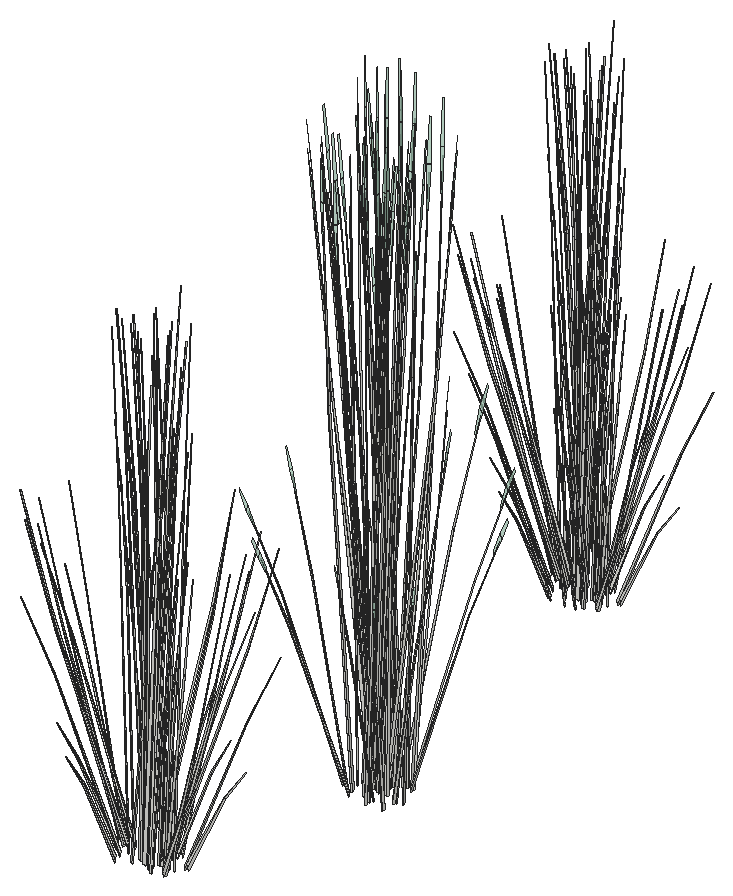
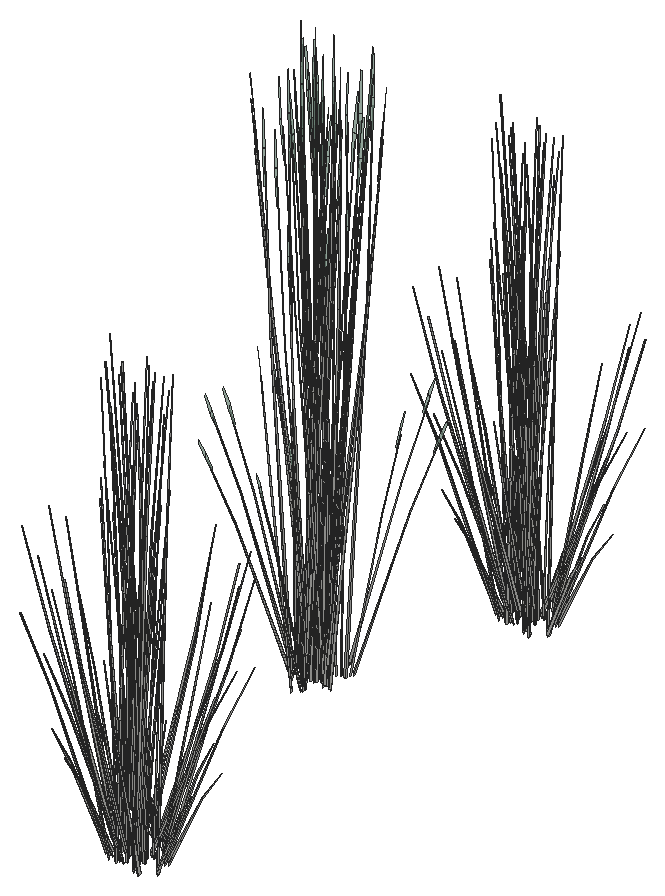
# SketchUp Ruby script. Lengths in inches.
U = 1.inch
M = Sketchup.active_model
def pt(a) = Geom::Point3d.new(a.map { |v| v * U })
def face(e, loops, mat)
  f = e.add_face(loops[0].map { |a| pt(a) })
  loops[1..].each { |l| e.add_face(l.map { |a| pt(a) }).erase! }
  f.material = f.back_material = mat if mat
  f
end
# faces: each face lists its corners as indices into pts; further lists are holes
def faces(e, pts, list, mat = nil) = list.each { |f| face(e, (f[0].is_a?(Array) ? f : [f]).map { |l| l.map { |i| pts[i] } }, mat) }
# xy, xz, yz: faces in a plane at the given z, y or x. An outline is a flat list of corners, or four numbers for a rectangle; further outlines are holes
def ring(l) = l.size == 4 ? [[l[0], l[1]], [l[2], l[1]], [l[2], l[3]], [l[0], l[3]]] : l.each_slice(2).to_a
def flat(e, list, mat, &to3) = list.each { |f| face(e, (f[0].is_a?(Array) ? f : [f]).map { |l| ring(l).map { |u, v| to3.(u, v) } }, mat) }
def xy(e, z, list, mat = nil) = flat(e, list, mat) { |x, y| [x, y, z] }
def xz(e, y, list, mat = nil) = flat(e, list, mat) { |x, z| [x, y, z] }
def yz(e, x, list, mat = nil) = flat(e, list, mat) { |y, z| [x, y, z] }
def lines(e, pts, list) = list.each { |a, b| e.add_line(pt(pts[a]), pt(pts[b])) }
# prism: a flat outline (further loops are holes) pulled along v
def prism(e, loops, v, mat = nil)
  f = face(e, loops, mat); d = Geom::Vector3d.new(v.map { |x| x * U })
  f.pushpull(f.normal.samedirection?(d) ? d.length : -d.length)
end
def box(e, o, s, mat = nil) = prism(e, [[o, [o[0] + s[0], o[1], o[2]], [o[0] + s[0], o[1] + s[1], o[2]], [o[0], o[1] + s[1], o[2]]]], [0, 0, s[2]], mat)
def at(x, y, z, deg = 0) = Geom::Transformation.translation(pt([x, y, z])) * Geom::Transformation.rotation(ORIGIN, Z_AXIS, deg.degrees)
def axes(o, x, y, z) = Geom::Transformation.new([*x, 0, *y, 0, *z, 0, *pt(o).to_a, 1])
def part(name) = M.definitions.add(name)
# library, detail: a bought-in or finely detailed component or shape, given as its bounding box
def library(name, o, s) = part(name).tap { |d| box(d.entities, o, s) }
def detail(e, o, s) = box(e.add_group.entities, o, s)
def put(e, d, t, mat = nil) = e.add_instance(d, t).tap { |i| i.material = mat if mat }
def group(e, t, mat = nil) = e.add_group.tap { |g| g.transformation = t; g.material = mat if mat }.entities
root = M.entities
M.materials.add("LightPink_Translucent").color = [175, 214, 192]
M.materials["LightPink_Translucent"].alpha = 0.75
c1 = part("blade")
p = [[2.15,0.21,22],[0,0.17,0],[0.09,0.45,0],[2.18,0.31,22],[2.29,0.31,22],[0.38,0.45,0],
  [2.48,0.24,33],[2.49,0.24,33],[2.48,0.22,33]]
faces(c1.entities,p,[[0,1,2,3],[4,5,2,3],[6,3,4,7],[8,0,3,6]])
c2 = part("blade with seeds\#1")
put(c2.entities,c1,at(0,0,0))
c3 = part("seeds")
p = [[0.3,-0.1,1.38],[-0.01,-0.03,1.59],[-0.01,-0.03,0.03],[0.14,-0.07,-0.07],[0.29,-0.03,3],[0.15,0.01,3.11]]
faces(c3.entities,p,[[0,1,2,3],[1,0,4,5]],"LightPink_Translucent")
c4 = part("blade with seeds")
put(c4.entities,c1,at(0,0,0))
put(c4.entities,c3,axes([2.4,0.25,30.99],[1.5799,-0.05474,1.17369],[-0.12525,1.92788,0.29478],[-0.07173,-0.02425,1.56792]))
put(root,c2,axes([484.73,498.58,138.99],[0.25932,0.13262,0.94226],[-0.37767,0.07972,0.69231],[-0.08081,-0.10192,0.20754]))
put(root,c2,axes([485.36,499.28,140.8],[-0.4239,-0.18418,-0.58282],[0.30126,-0.32274,0.07033],[-0.15358,-0.10997,0.82446]))
put(root,c2,axes([485.16,499.29,140.56],[-0.49056,0.09058,-0.41919],[-0.08581,-0.34303,-0.3247],[-0.13176,-0.0983,0.80208]))
put(root,c2,axes([488.05,499.97,140.56],[-0.12771,-0.34793,-0.41919],[0.48364,-0.06086,-0.3247],[0.1386,-0.09345,0.80208]))
put(root,c2,axes([488.06,500.11,140.8],[0.25968,-0.30066,-0.58282],[0.45504,0.21367,0.07033],[0.15505,-0.10893,0.82446]))
put(root,c2,axes([488.43,499.84,138.84],[-0.1776,-0.01129,1.17311],[-0.18194,-0.30276,-0.25229],[0.21818,-0.08565,0.50157]))
put(root,c2,axes([488.64,499.28,138.99],[-0.16559,0.19397,0.94226],[-0.14233,-0.26061,0.69231],[0.13676,-0.0653,0.20754]))
put(root,c2,axes([484.09,499.83,138.84],[0.09706,0.10609,1.17311],[-0.22366,0.28837,-0.25229],[-0.22965,-0.06892,0.50157]))
put(root,c2,axes([484.5,499.74,140.8],[-0.49695,-0.00917,-0.58282],[0.03338,-0.38634,0.07033],[-0.21053,-0.04077,0.82446]))
put(root,c2,axes([484.33,499.82,140.56],[-0.36098,0.25241,-0.41919],[-0.31614,-0.26664,-0.3247],[-0.18341,-0.0384,0.80208]))
put(root,c2,axes([485.94,500.63,138.71],[0.56014,0.18468,0.19741],[-0.26958,0.38374,0.41019],[0,-0.08846,1.31701]))
put(root,c2,axes([483.52,500.15,138.99],[0.31739,-0.02727,0.94226],[-0.20133,0.24024,0.69231],[-0.15684,-0.03604,0.20754]))
put(root,c2,axes([485.76,500.375,138.95],[-0.53984,0.02352,0.36702],[-0.04882,-0.39046,-0.17663],[0.09664,-0.03957,1.17838]))
put(root,c2,axes([484.37,500.66,138.75],[0,0.38104,0.40731],[-0.5562,0,0],[0,-0.08679,1.29208]))
put(root,c2,axes([485.74,500.52,138.65],[0.21614,0.42608,0.37535],[-0.61757,0.14817,0.14729],[0.00755,-0.07829,1.30318]))
put(root,c2,axes([488.27,500.74,140.56],[0.13468,-0.34661,-0.41919],[0.46175,0.1188,-0.3247],[0.18591,-0.03178,0.80208]))
put(root,c2,axes([487.27,499.53,138.75],[-0.46527,-0.19052,0.40731],[0.2781,-0.34163,0],[0.10597,0.04339,1.29208]))
put(root,c2,axes([485.63,500.85,138.95],[-0.2412,0.34335,0.36702],[-0.50118,-0.16524,-0.17663],[0,-0.07915,1.17838]))
put(root,c2,axes([486.22,500.27,138.65],[-0.41219,0.3458,0.37535],[-0.4897,-0.30525,0.14729],[0.09937,-0.03451,1.30318]))
put(root,c2,axes([485.51,499.7,138.75],[-0.14361,0.37869,0.14473],[-0.52552,-0.10717,0.28783],[0.09078,-0.00184,1.3159]))
put(root,c2,axes([488.18,500.87,140.8],[0.43684,-0.16829,-0.58282],[0.24345,0.34641,0.07033],[0.21107,-0.03935,0.82446]))
put(root,c2,axes([486.61,500.125,138.86],[0.0959,-0.34006,0.11878],[0.46856,0.05903,-0.33919],[0.08527,0.03492,1.03975]))
put(root,c2,axes([486.41,500.21,138.95],[-0.29864,-0.31983,0.36702],[0.45236,-0.22522,-0.17663],[0.09664,0.03957,1.17838]))
put(root,c2,axes([485.8,500.93,138.65],[0.62833,0.08028,0.37535],[-0.12787,0.45342,0.14729],[-0.09182,-0.04378,1.30318]))
put(root,c2,axes([487.1,499.72,138.75],[-0.5342,0.10113,0.14473],[-0.13191,-0.37638,0.28783],[0.04764,0.05484,1.3159]))
put(root,c2,axes([485.46,501.66,138.75],[0.5342,-0.10113,0.14473],[0.13191,0.37638,0.28783],[-0.04764,-0.05484,1.3159]))
put(root,c2,axes([486.76,500.45,138.67],[-0.62833,-0.08028,0.4036],[0.12787,-0.45342,0.15838],[0.09182,0.04378,1.40127]))
put(root,c2,axes([485.95,501.26,138.86],[-0.0959,0.34006,0.11878],[-0.46856,-0.05903,-0.33919],[-0.08527,-0.03492,1.03975]))
put(root,c2,axes([487.87,500.71,138.75],[-0.39059,-0.27756,0.14473],[0.39362,-0.26921,0.28783],[-0.04314,0.05668,1.3159]))
put(root,c2,axes([484.96,500.36,139.46],[0.14131,-0.05512,1.45254],[0.04873,0.38487,0.11368],[-0.30608,0.05107,0.51915]))
put(root,c2,axes([489.43,500.97,138.99],[-0.30716,0.06291,0.94226],[0.14458,-0.25998,0.69231],[0.16295,0.01779,0.20754]))
put(root,c2,axes([487.05,501.68,138.75],[0.14361,-0.37869,0.14473],[0.52552,0.10717,0.28783],[-0.09078,0.00184,1.3159]))
put(root,c2,axes([486.92,500.53,138.95],[0.2412,-0.34335,0.36702],[0.50118,0.16524,-0.17663],[0,0.07915,1.17838]))
put(root,c2,axes([485.28,501.85,138.75],[0.46527,0.19052,0.40731],[-0.2781,0.34163,0],[-0.10597,-0.04339,1.29208]))
put(root,c2,axes([483.98,500.57,140.56],[-0.13468,0.34661,-0.41919],[-0.46175,-0.1188,-0.3247],[-0.18591,0.03178,0.80208]))
put(root,c2,axes([488.1875,500.72,138.75],[0,-0.38104,0.40731],[0.5562,0,0],[0,0.08679,1.29208]))
put(root,c2,axes([487.13,500.61,138.86],[0.46318,-0.11112,0.11878],[0.1622,0.31732,-0.33919],[0,0.06984,1.03975]))
put(root,c2,axes([486.8,501.01,138.95],[0.53984,-0.02352,0.36702],[0.04882,0.39046,-0.17663],[-0.09664,0.03957,1.17838]))
put(root,c2,axes([488.85,501.38,138.84],[-0.11973,-0.09372,1.17311],[0.15578,-0.31002,-0.25229],[0.24224,0.042,0.50157]))
put(root,c2,axes([486.8,501.18,138.86],[0.36728,0.22894,0.11878],[-0.30636,0.25829,-0.33919],[-0.08527,0.03492,1.03975]))
put(root,c2,axes([487.76,501.57,140.8],[0.49695,0.00917,-0.58282],[-0.03338,0.38634,0.07033],[0.21053,0.04077,0.82446]))
put(root,c2,axes([487.2,501.88,138.75],[0.46527,-0.19052,0.40731],[0.2781,0.34163,0],[-0.10597,0.04339,1.29208]))
put(root,c2,axes([483.43,501.38,138.84],[0.17277,0.03128,1.17311],[0.11135,0.3195,-0.25229],[-0.23468,0.05981,0.50157]))
put(root,c2,axes([483.07,502.05,138.99],[0.20718,-0.1727,0.94226],[0.08175,0.27339,0.69231],[-0.14972,0.04895,0.20754]))
put(root,c2,axes([487.72,501.87,138.99],[-0.27991,-0.10956,0.94226],[0.36143,-0.11132,0.69231],[0.09749,0.0943,0.20754]))
put(root,c2,axes([484.21,501.34,140.56],[0.12771,0.34793,-0.41919],[-0.48364,0.06086,-0.3247],[-0.1386,0.09345,0.80208]))
put(root,c2,axes([487.04,500.63,139.05],[-0.01358,-0.35877,1.15892],[0.61462,0.093,0.4907],[-0.14537,0.19631,1.09393]))
put(root,c2,axes([487.09,502.02,140.56],[0.49056,-0.09058,-0.41919],[0.08581,0.34303,-0.3247],[0.13176,0.0983,0.80208]))
put(root,c2,axes([487.77,502.37,138.91],[-0.31879,-0.01195,0.86186],[0.21053,-0.25381,0.47585],[0.12594,0.09017,0.67605]))
put(root,c2,axes([486.73,501.75,138.84],[0.00877,-0.12631,1.17311],[0.41923,-0.14109,-0.25229],[0.12942,0.15118,0.50157]))
put(root,c2,axes([484.82,502.8,138.99],[-0.01287,-0.22657,0.94226],[0.32149,0.1616,0.69231],[-0.06323,0.10799,0.20754]))
put(root,c2,axes([486,502.18,140.56],[0.48869,0.09552,-0.41919],[-0.16751,0.3275,-0.3247],[0.04481,0.13186,0.80208]))
put(root,c2,axes([484.56,502.3125,139.03],[0.45162,-0.06748,0.05338],[0.10383,0.27185,-0.708],[-0.02863,0.13761,0.63462]))
put(root,c2,axes([484.83,501.8125,141.1],[-0.01294,0.35246,-0.64693],[-0.54471,-0.02367,0.07807],[-0.05748,0.14932,0.91515]))
put(root,c2,axes([485.82,502.11,140.8],[0.23727,0.30983,-0.58282],[-0.48842,0.17267,0.07033],[0.05548,0.1497,0.82446]))
put(root,c2,axes([484.45,502.6,138.84],[0.15688,-0.06011,1.17311],[0.38733,0.18125,-0.25229],[-0.11528,0.15683,0.50157]))
put(root,c4,axes([492.18,515.8,139.53],[-0.03656,0.1661,1.30132],[-0.37341,0.10705,-0.27986],[-0.0699,-0.22562,0.55638]))
put(root,c4,axes([493.98,516.4375,139.53],[-0.12399,0.09331,1.30132],[-0.33702,-0.21502,-0.27986],[0.08055,-0.22079,0.55638]))
put(root,c4,axes([491.39,517.32,139.33],[-0.44625,-0.29882,0],[0.24886,-0.49993,-0.46963],[0.05668,-0.11386,1.48977]))
put(root,c4,axes([490.75,516.78,139.53],[0.07025,0.15082,1.30132],[-0.21183,0.37238,-0.27986],[-0.18329,-0.11083,0.55638]))
put(root,c4,axes([494.75,516.56,139.11],[-0.36364,-0.13787,-0.03542],[0.11186,-0.42434,-0.16061],[0.05948,-0.06443,0.52975]))
put(root,c4,axes([495.21,517.2,139.53],[-0.14568,-0.02894,1.30132],[-0.12195,-0.4231,-0.27986],[0.1883,-0.0989,0.55638]))
put(root,c4,axes([492.45,518.27,139.6],[-0.29566,-0.48255,-0.26477],[0.41776,-0.32089,-0.45502],[0.04243,-0.11906,1.45334]))
put(root,c4,axes([493.09,516.34,139.33],[0,-0.59763,0],[0.49772,0,-0.46963],[0.11336,0,1.48977]))
put(root,c4,axes([493.23,516.8,139.29],[-0.37441,-0.44456,0.27988],[0.37047,-0.44483,-0.33208],[0.10632,-0.01552,1.50045]))
put(root,c4,axes([492.3125,518.81,139.41],[0.35844,-0.4667,-0.22925],[0.40249,0.39271,0.50168],[-0.04193,-0.12567,1.53076]))
put(root,c4,axes([491.63,517.58,139.43],[-0.22267,0.44731,0.45182],[-0.39927,-0.26736,0],[0.05071,-0.10188,1.43328]))
put(root,c4,axes([492.44,518,139.39],[0.5277,0.12668,-0.2132],[-0.09198,0.60063,0.46656],[0.07287,-0.10495,1.42361]))
put(root,c4,axes([492.32,518.22,139.55],[-0.39744,-0.0922,0.13176],[0.06899,-0.45047,-0.37626],[0.04081,-0.08198,1.15337]))
put(root,c4,axes([493.02,516.7,139.43],[-0.44533,0,0.45182],[0,-0.53472,0],[0.10143,0,1.43328]))
put(root,c4,axes([491.33,519.15,139.17],[0.44781,-0.29509,-0.04679],[0.24886,0.49993,0.46963],[-0.04264,-0.12319,1.48904]))
put(root,c4,axes([492.92,517.87,139.6],[0.21249,-0.53825,-0.26477],[0.44849,0.25917,-0.45502],[0.11011,-0.01692,1.45334]))
put(root,c4,axes([491.09,516.88,139.74],[0.07886,0.43418,0.05922],[-0.31771,0.09982,-0.78537],[-0.16083,-0.02753,0.70398]))
put(root,c4,axes([492.51,518.9375,139.6],[-0.50815,0.05569,-0.26477],[-0.03072,-0.58006,-0.45502],[-0.06769,-0.10214,1.45334]))
put(root,c4,axes([495.22,518.21,139.11],[-0.25548,-0.33028,-0.03542],[0.27981,-0.30262,-0.16061],[0.07928,-0.02131,0.52975]))
put(root,c4,axes([492.7,518.07,139.32],[-0.09383,0.60408,0.41637],[-0.52992,-0.12294,0.16339],[0.05117,-0.08828,1.44559]))
put(root,c4,axes([491.85,517.75,139.42],[0.1182,0.51358,0.16054],[-0.43988,0.12682,0.31929],[0.06409,-0.0458,1.4597]))
put(root,c4,axes([491.78,518.41,139.17],[0.19993,-0.48183,0],[0.41543,0.23189,0],[0,0,1.48063]))
put(root,c4,axes([491.28,519.53,139.33],[-0.44625,0.29882,0],[-0.24886,-0.49993,-0.46963],[-0.05668,-0.11386,1.48977]))
put(root,c4,axes([491.83,519.28,139.42],[0.44258,0.13807,0.16054],[-0.12525,0.50524,0.31929],[-0.00216,-0.08728,1.4597]))
put(root,c4,axes([492.42,519.04,139.55],[-0.26757,0.3531,0.13176],[-0.30187,-0.29453,-0.37626],[-0.04081,-0.08198,1.15337]))
put(root,c4,axes([492.75,518.92,139.26],[0.3833,-0.44456,-0.05579],[0.38354,0.44483,0],[0.01339,-0.01552,1.5977]))
put(root,c4,axes([491.5625,519.16,139.29],[-0.14475,0.59835,0.27988],[-0.51739,-0.14969,-0.33208],[-0.06475,-0.09903,1.50045]))
put(root,c4,axes([491.59,519.42,139.43],[0.22267,0.44731,0.45182],[-0.39927,0.26736,0],[-0.05071,-0.10188,1.43328]))
put(root,c4,axes([493.1875,518.02,139.32],[-0.49797,0.2078,0.41637],[-0.17316,-0.59373,0.16339],[0.0915,0.00726,1.44559]))
put(root,c4,axes([491.96,518.52,139.18],[0.38394,-0.15594,0],[0.13445,0.4453,0],[0,0,1.40478]))
put(root,c4,axes([492.96,520.07,139.42],[0.32439,-0.37551,0.16054],[0.31463,0.37842,0.31929],[-0.06625,-0.04147,1.4597]))
put(root,c4,axes([493.14,518.77,139.18],[0.51528,0,0],[0,0.59763,0],[0,0,1.63305]))
put(root,c4,axes([493.05,518.21,139.38],[-0.21584,0.53851,0.21899],[-0.44849,-0.25917,0.45502],[0.10338,0,1.46094]))
put(root,c4,axes([492.9375,519.07,139.26],[-0.51503,0,-0.0513],[0,-0.59763,0],[-0.01619,0,1.63225]))
put(root,c4,axes([494.13,517.8,139.42],[-0.44258,-0.13807,0.16054],[0.12525,-0.50524,0.31929],[0.00216,0.08728,1.4597]))
put(root,c4,axes([491.94,518.78,139.25],[-0.51161,0.2078,-0.05471],[-0.17927,-0.59373,0],[-0.01787,0.00726,1.56677]))
put(root,c4,axes([494.68,517.55,139.33],[0.44625,-0.29882,0],[0.24886,0.49993,-0.46963],[0.05668,0.11386,1.48977]))
put(root,c4,axes([492.61,520.5,139.17],[0.00356,-0.59734,-0.04529],[0.49772,0,0.45448],[-0.1133,-0.01877,1.441]))
put(root,c4,axes([494.11,519.33,139.42],[-0.1182,-0.51358,0.16054],[0.43988,-0.12682,0.31929],[-0.06409,0.0458,1.4597]))
put(root,c4,axes([493.47,518.49,139.32],[-0.40415,-0.39628,0.41637],[0.35675,-0.4708,0.16339],[0.04033,0.09554,1.44559]))
put(root,c4,axes([492.83,519.16,139.19],[-0.28765,0.33362,0],[-0.28765,-0.33362,0],[0,0,1.54032]))
put(root,c4,axes([491.77,518.96,139.18],[-0.19993,0.48183,0],[-0.41543,-0.23189,0],[0,0,1.59208]))
put(root,c4,axes([493.26,519,139.34],[0.09383,-0.60408,0.44771],[0.52992,0.12294,0.17569],[-0.05117,0.08828,1.5544]))
put(root,c4,axes([493.03,519.17,139.18],[0,0.53472,0],[-0.46104,0,0],[0,0,1.6235]))
put(root,c4,axes([493.45,518.14,139.6],[0.50815,-0.05569,-0.26477],[0.03072,0.58006,-0.45502],[0.06769,0.10214,1.45334]))
put(root,c4,axes([493.08,519.36,139.55],[0.12987,0.4453,0.13176],[-0.37086,0.15594,-0.37626],[-0.08162,0,1.15337]))
put(root,c4,axes([493.05,519.21,139.6],[-0.21249,0.53825,-0.26477],[-0.44849,-0.25917,-0.45502],[-0.11011,0.01692,1.45334]))
put(root,c4,axes([495.04,519.3,139.53],[-0.09014,-0.13585,1.30132],[0.15777,-0.40687,-0.27986],[0.19621,0.07542,0.55638]))
put(root,c4,axes([492.94,520.375,139.43],[0.44533,0,0.45182],[0,0.53472,0],[-0.10143,0,1.43328]))
put(root,c4,axes([493.64,518.85,139.55],[0.39744,0.0922,0.13176],[-0.06899,0.45047,-0.37626],[-0.04081,0.08198,1.15337]))
put(root,c4,axes([494.34,519.49,139.43],[0.22267,-0.44731,0.45182],[0.39927,0.26736,0],[-0.05071,0.10188,1.43328]))
put(root,c4,axes([492.01,519.1,139.16],[0.1511,0.50177,-0.1747],[-0.43526,0.17632,0.00007],[0.0167,0.05539,1.58246]))
put(root,c4,axes([491.74,518.97,139.53],[0.14762,0.00843,1.30132],[0.1649,0.40305,-0.27986],[-0.17669,0.12442,0.55638]))
put(root,c4,axes([492.87,520.74,139.33],[0,0.59763,0],[-0.49772,0,-0.46963],[-0.11336,0,1.48977]))
put(root,c4,axes([493.51,518.81,139.6],[0.29566,0.48255,-0.26477],[-0.41776,0.32089,-0.45502],[-0.04243,0.11906,1.45334]))
put(root,c4,axes([494.57,519.75,139.33],[0.44625,0.29882,0],[-0.24886,0.49993,-0.46963],[-0.05668,0.11386,1.48977]))
put(root,c4,axes([493.18,521.49,139.23],[0.28477,-0.29631,-0.05904],[0.26092,0.32453,-0.26768],[0.01837,0.09195,0.88292]))
put(root,c4,axes([493.98,520.61,139.53],[0.01319,-0.17074,1.30132],[0.35385,-0.17492,-0.27986],[0.1001,0.20976,0.55638]))
put(root,c4,axes([492.8,520.93,138.97],[-0.05344,-0.30783,1.28841],[0.4254,-0.049,0.07375],[0.06439,0.2156,0.73315]))
put(root,c4,axes([492.17,521.01,139.53],[0.10953,-0.1151,1.30132],[0.36232,0.14976,-0.27986],[-0.04908,0.23288,0.55638]))
put(root,c2,axes([487.07,547.98,138.84],[-0.14131,0.07713,1.17311],[-0.4232,-0.13499,-0.25229],[0.07845,-0.16789,0.50157]))
put(root,c2,axes([486.43,548.25,140.8],[-0.23727,-0.30983,-0.58282],[0.48842,-0.17267,0.07033],[-0.05548,-0.1497,0.82446]))
put(root,c2,axes([484.89,547.83,138.84],[-0.0301,0.12465,1.17311],[-0.44009,0.10435,-0.25229],[-0.10287,-0.16111,0.50157]))
put(root,c2,axes([487.42,548.55,140.8],[0.01294,-0.35246,-0.58282],[0.54471,0.02367,0.07033],[0.05748,-0.14932,0.82446]))
put(root,c2,axes([486.55,547.36,138.99],[0.06377,0.2222,0.94226],[-0.35378,-0.12306,0.69231],[0.03807,-0.11377,0.20754]))
put(root,c2,axes([486.25,548.18,140.56],[-0.48869,-0.09552,-0.41919],[0.16751,-0.3275,-0.3247],[-0.04481,-0.13186,0.80208]))
put(root,c2,axes([487.31,548.43,140.56],[-0.35588,-0.25603,-0.41919],[0.37594,-0.22422,-0.3247],[0.05415,-0.13008,0.80208]))
put(root,c2,axes([484.73,547.63,138.99],[0.25932,0.13262,0.94226],[-0.37767,0.07972,0.69231],[-0.08081,-0.10192,0.20754]))
put(root,c2,axes([485.36,548.33,140.8],[-0.4239,-0.18418,-0.58282],[0.30126,-0.32274,0.07033],[-0.15358,-0.10997,0.82446]))
put(root,c2,axes([485.16,548.34,140.56],[-0.49056,0.09058,-0.41919],[-0.08581,-0.34303,-0.3247],[-0.13176,-0.0983,0.80208]))
put(root,c2,axes([488.05,549.02,140.56],[-0.12771,-0.34793,-0.41919],[0.48364,-0.06086,-0.3247],[0.1386,-0.09345,0.80208]))
put(root,c2,axes([488.06,549.16,140.8],[0.25968,-0.30066,-0.58282],[0.45504,0.21367,0.07033],[0.15505,-0.10893,0.82446]))
put(root,c2,axes([488.43,548.88,138.84],[-0.1776,-0.01129,1.17311],[-0.18194,-0.30276,-0.25229],[0.21818,-0.08565,0.50157]))
put(root,c2,axes([488.64,548.33,138.99],[-0.16559,0.19397,0.94226],[-0.14233,-0.26061,0.69231],[0.13676,-0.0653,0.20754]))
put(root,c2,axes([484.09,548.88,138.84],[0.09706,0.10609,1.17311],[-0.22366,0.28837,-0.25229],[-0.22965,-0.06892,0.50157]))
put(root,c2,axes([484.5,548.79,140.8],[-0.49695,-0.00917,-0.58282],[0.03338,-0.38634,0.07033],[-0.21053,-0.04077,0.82446]))
put(root,c2,axes([484.33,548.87,140.56],[-0.36098,0.25241,-0.41919],[-0.31614,-0.26664,-0.3247],[-0.18341,-0.0384,0.80208]))
put(root,c2,axes([485.94,549.68,138.71],[0.56014,0.18468,0.19741],[-0.26958,0.38374,0.41019],[0,-0.08846,1.31701]))
put(root,c2,axes([483.52,549.2,138.99],[0.31739,-0.02727,0.94226],[-0.20133,0.24024,0.69231],[-0.15684,-0.03604,0.20754]))
put(root,c2,axes([485.76,549.42,138.95],[-0.53984,0.02352,0.36702],[-0.04882,-0.39046,-0.17663],[0.09664,-0.03957,1.17838]))
put(root,c2,axes([484.37,549.71,138.75],[0,0.38104,0.40731],[-0.5562,0,0],[0,-0.08679,1.29208]))
put(root,c2,axes([485.74,549.5625,138.65],[0.21614,0.42608,0.37535],[-0.61757,0.14817,0.14729],[0.00755,-0.07829,1.30318]))
put(root,c2,axes([488.27,549.79,140.56],[0.13468,-0.34661,-0.41919],[0.46175,0.1188,-0.3247],[0.18591,-0.03178,0.80208]))
put(root,c2,axes([487.27,548.58,138.75],[-0.46527,-0.19052,0.40731],[0.2781,-0.34163,0],[0.10597,0.04339,1.29208]))
put(root,c2,axes([485.63,549.9,138.95],[-0.2412,0.34335,0.36702],[-0.50118,-0.16524,-0.17663],[0,-0.07915,1.17838]))
put(root,c2,axes([486.22,549.32,138.65],[-0.41219,0.3458,0.37535],[-0.4897,-0.30525,0.14729],[0.09937,-0.03451,1.30318]))
put(root,c2,axes([485.51,548.75,138.75],[-0.14361,0.37869,0.14473],[-0.52552,-0.10717,0.28783],[0.09078,-0.00184,1.3159]))
put(root,c2,axes([488.18,549.92,140.8],[0.43684,-0.16829,-0.58282],[0.24345,0.34641,0.07033],[0.21107,-0.03935,0.82446]))
put(root,c2,axes([486.61,549.17,138.86],[0.0959,-0.34006,0.11878],[0.46856,0.05903,-0.33919],[0.08527,0.03492,1.03975]))
put(root,c2,axes([486.41,549.26,138.95],[-0.29864,-0.31983,0.36702],[0.45236,-0.22522,-0.17663],[0.09664,0.03957,1.17838]))
put(root,c2,axes([485.8,549.98,138.65],[0.62833,0.08028,0.37535],[-0.12787,0.45342,0.14729],[-0.09182,-0.04378,1.30318]))
put(root,c2,axes([487.1,548.77,138.75],[-0.5342,0.10113,0.14473],[-0.13191,-0.37638,0.28783],[0.04764,0.05484,1.3159]))
put(root,c2,axes([485.46,550.71,138.75],[0.5342,-0.10113,0.14473],[0.13191,0.37638,0.28783],[-0.04764,-0.05484,1.3159]))
put(root,c2,axes([486.76,549.5,138.67],[-0.62833,-0.08028,0.4036],[0.12787,-0.45342,0.15838],[0.09182,0.04378,1.40127]))
put(root,c2,axes([485.95,550.31,138.86],[-0.0959,0.34006,0.11878],[-0.46856,-0.05903,-0.33919],[-0.08527,-0.03492,1.03975]))
put(root,c2,axes([487.87,549.76,138.75],[-0.39059,-0.27756,0.14473],[0.39362,-0.26921,0.28783],[-0.04314,0.05668,1.3159]))
put(root,c2,axes([484.96,549.41,139.46],[0.14131,-0.05512,1.45254],[0.04873,0.38487,0.11368],[-0.30608,0.05107,0.51915]))
put(root,c2,axes([489.43,550.01,138.99],[-0.30716,0.06291,0.94226],[0.14458,-0.25998,0.69231],[0.16295,0.01779,0.20754]))
put(root,c2,axes([487.05,550.73,138.75],[0.14361,-0.37869,0.14473],[0.52552,0.10717,0.28783],[-0.09078,0.00184,1.3159]))
put(root,c2,axes([486.92,549.58,138.95],[0.2412,-0.34335,0.36702],[0.50118,0.16524,-0.17663],[0,0.07915,1.17838]))
put(root,c2,axes([485.28,550.9,138.75],[0.46527,0.19052,0.40731],[-0.2781,0.34163,0],[-0.10597,-0.04339,1.29208]))
put(root,c2,axes([483.98,549.62,140.56],[-0.13468,0.34661,-0.41919],[-0.46175,-0.1188,-0.3247],[-0.18591,0.03178,0.80208]))
put(root,c2,axes([488.1875,549.77,138.75],[0,-0.38104,0.40731],[0.5562,0,0],[0,0.08679,1.29208]))
put(root,c2,axes([487.13,549.66,138.86],[0.46318,-0.11112,0.11878],[0.1622,0.31732,-0.33919],[0,0.06984,1.03975]))
put(root,c2,axes([486.8,550.06,138.95],[0.53984,-0.02352,0.36702],[0.04882,0.39046,-0.17663],[-0.09664,0.03957,1.17838]))
put(root,c2,axes([488.85,550.43,138.84],[-0.11973,-0.09372,1.17311],[0.15578,-0.31002,-0.25229],[0.24224,0.042,0.50157]))
put(root,c2,axes([486.8,550.22,138.86],[0.36728,0.22894,0.11878],[-0.30636,0.25829,-0.33919],[-0.08527,0.03492,1.03975]))
put(root,c2,axes([487.76,550.62,140.8],[0.49695,0.00917,-0.58282],[-0.03338,0.38634,0.07033],[0.21053,0.04077,0.82446]))
put(root,c2,axes([487.2,550.93,138.75],[0.46527,-0.19052,0.40731],[0.2781,0.34163,0],[-0.10597,0.04339,1.29208]))
put(root,c2,axes([483.43,550.43,138.84],[0.17277,0.03128,1.17311],[0.11135,0.3195,-0.25229],[-0.23468,0.05981,0.50157]))
put(root,c2,axes([483.07,551.1,138.99],[0.20718,-0.1727,0.94226],[0.08175,0.27339,0.69231],[-0.14972,0.04895,0.20754]))
put(root,c2,axes([487.72,550.92,138.99],[-0.27991,-0.10956,0.94226],[0.36143,-0.11132,0.69231],[0.09749,0.0943,0.20754]))
put(root,c2,axes([484.21,550.39,140.56],[0.12771,0.34793,-0.41919],[-0.48364,0.06086,-0.3247],[-0.1386,0.09345,0.80208]))
put(root,c2,axes([487.04,549.68,139.05],[-0.01358,-0.35877,1.15892],[0.61462,0.093,0.4907],[-0.14537,0.19631,1.09393]))
put(root,c2,axes([487.09,551.07,140.56],[0.49056,-0.09058,-0.41919],[0.08581,0.34303,-0.3247],[0.13176,0.0983,0.80208]))
put(root,c2,axes([487.77,551.41,138.91],[-0.31879,-0.01195,0.86186],[0.21053,-0.25381,0.47585],[0.12594,0.09017,0.67605]))
put(root,c2,axes([486.73,550.8,138.84],[0.00877,-0.12631,1.17311],[0.41923,-0.14109,-0.25229],[0.12942,0.15118,0.50157]))
put(root,c2,axes([484.82,551.85,138.99],[-0.01287,-0.22657,0.94226],[0.32149,0.1616,0.69231],[-0.06323,0.10799,0.20754]))
put(root,c2,axes([486,551.23,140.56],[0.48869,0.09552,-0.41919],[-0.16751,0.3275,-0.3247],[0.04481,0.13186,0.80208]))
put(root,c2,axes([484.56,551.36,139.03],[0.45162,-0.06748,0.05338],[0.10383,0.27185,-0.708],[-0.02863,0.13761,0.63462]))
